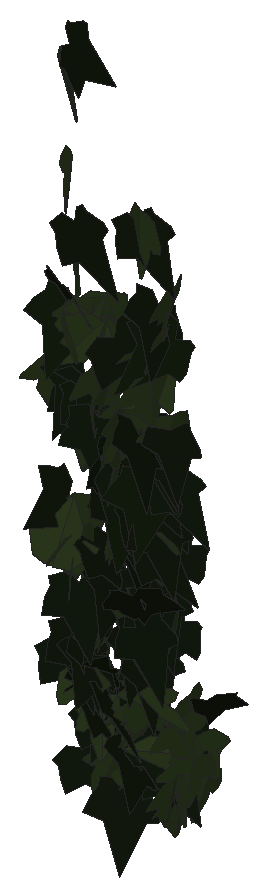
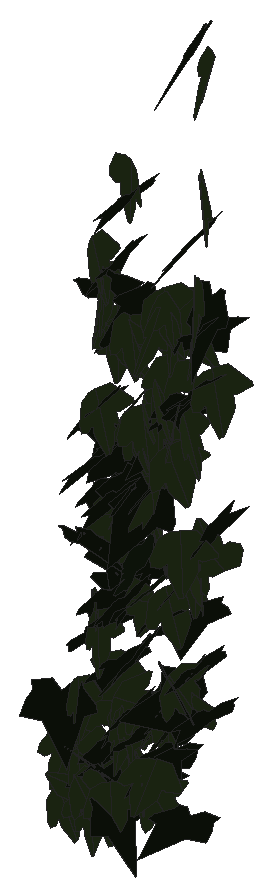
# SketchUp Ruby script. Lengths in inches.
U = 1.inch
M = Sketchup.active_model
def pt(a) = Geom::Point3d.new(a.map { |v| v * U })
def face(e, loops, mat)
  f = e.add_face(loops[0].map { |a| pt(a) })
  loops[1..].each { |l| e.add_face(l.map { |a| pt(a) }).erase! }
  f.material = f.back_material = mat if mat
  f
end
# faces: each face lists its corners as indices into pts; further lists are holes
def faces(e, pts, list, mat = nil) = list.each { |f| face(e, (f[0].is_a?(Array) ? f : [f]).map { |l| l.map { |i| pts[i] } }, mat) }
# xy, xz, yz: faces in a plane at the given z, y or x. An outline is a flat list of corners, or four numbers for a rectangle; further outlines are holes
def ring(l) = l.size == 4 ? [[l[0], l[1]], [l[2], l[1]], [l[2], l[3]], [l[0], l[3]]] : l.each_slice(2).to_a
def flat(e, list, mat, &to3) = list.each { |f| face(e, (f[0].is_a?(Array) ? f : [f]).map { |l| ring(l).map { |u, v| to3.(u, v) } }, mat) }
def xy(e, z, list, mat = nil) = flat(e, list, mat) { |x, y| [x, y, z] }
def xz(e, y, list, mat = nil) = flat(e, list, mat) { |x, z| [x, y, z] }
def yz(e, x, list, mat = nil) = flat(e, list, mat) { |y, z| [x, y, z] }
def lines(e, pts, list) = list.each { |a, b| e.add_line(pt(pts[a]), pt(pts[b])) }
# prism: a flat outline (further loops are holes) pulled along v
def prism(e, loops, v, mat = nil)
  f = face(e, loops, mat); d = Geom::Vector3d.new(v.map { |x| x * U })
  f.pushpull(f.normal.samedirection?(d) ? d.length : -d.length)
end
def box(e, o, s, mat = nil) = prism(e, [[o, [o[0] + s[0], o[1], o[2]], [o[0] + s[0], o[1] + s[1], o[2]], [o[0], o[1] + s[1], o[2]]]], [0, 0, s[2]], mat)
def at(x, y, z, deg = 0) = Geom::Transformation.translation(pt([x, y, z])) * Geom::Transformation.rotation(ORIGIN, Z_AXIS, deg.degrees)
def axes(o, x, y, z) = Geom::Transformation.new([*x, 0, *y, 0, *z, 0, *pt(o).to_a, 1])
def part(name) = M.definitions.add(name)
# library, detail: a bought-in or finely detailed component or shape, given as its bounding box
def library(name, o, s) = part(name).tap { |d| box(d.entities, o, s) }
def detail(e, o, s) = box(e.add_group.entities, o, s)
def put(e, d, t, mat = nil) = e.add_instance(d, t).tap { |i| i.material = mat if mat }
def group(e, t, mat = nil) = e.add_group.tap { |g| g.transformation = t; g.material = mat if mat }.entities
root = M.entities
M.materials.add("efeu1").color = [18, 25, 13]
M.materials.add("efeu2").color = [43, 57, 29]
c1 = part("ivyleaf_9")
p = [[1.54,2.16,1.25],[1.36,2.04,1.19],[-0.21,0.99,0.68],[-0.71,1.11,0.82],[-0.85,0.86,0.67],[-0.8,0.17,0.21],
  [-0.9,-0.01,0.1],[-0.67,-0.16,-0.02],[-0.08,-0.08,-0.05],[-0.03,-0.6,-0.4],[0.65,-0.88,-0.66],[0.83,-0.6,-0.49],
  [1.29,-0.42,-0.43],[1.8125,-0.07,-0.26],[1.21,0.44,0.15]]
faces(c1.entities,p,[[0,1,2,3,4,5,6,7,8,9,10,11,12,13,14]],"efeu1")
c2 = part("ivyleaf_10")
p = [[0,0.5,-0.03],[-0.0625,2.02,-0.43],[-0.19,2.01,-0.46],[-0.54,1.05,-0.29],[-0.52,0.625,-0.18],[-0.83,0.76,-0.28],
  [-1.16,0.64,-0.33],[-1.15,0.33,-0.24],[-0.77,-0.39,0.02],[-0.3,-0.51,0.16],[0.04,-0.48,0.23],[-0.02,2.01,-0.4375],
  [-0.06,2.01,-0.43],[0.04,-0.49,0.23],[0.67,-0.49,0.14],[1.38,0.36,-0.2],[1.375,0.51,-0.24],[0.81,0.65,-0.19],
  [0.62,0.59,-0.15],[0.6,1.09,-0.28],[0.5,1.23,-0.31]]
faces(c2.entities,p,[[0,1,2,3,4,5,6,7,8,9,10],[11,12,0,13,14,15,16,17,18,19,20]],"efeu2")
put(root,c1,axes([523.03,133.5,210.82],[0.21573,-0.75981,-0.367],[0.08957,0.39729,-0.76985],[0.83903,0.15295,0.17655]))
put(root,c2,axes([523.63,132.39,222.53],[-0.3306,-0.85871,0.06277],[-0.02819,-0.05641,-0.92013],[0.86054,-0.33174,-0.00602]))
put(root,c1,axes([523.49,133.05,216.98],[-0.21291,-0.48592,0.71831],[-0.21885,-0.6856,-0.52866],[0.83917,-0.30209,0.04437]))
put(root,c1,axes([523.875,132.32,225.51],[0.71123,0.0971,-0.62296],[-0.62829,0.0309,-0.7125],[-0.05254,0.94497,0.08731]))
put(root,c2,axes([523.84,133.06,226.16],[0.60515,-0.59939,-0.36822],[-0.0232,0.46845,-0.80067],[0.70308,0.53136,0.29052]))
put(root,c2,axes([523.79,132.78,229.89],[0.63105,-0.68924,-0.10856],[0.05514,0.19517,-0.91865],[0.69555,0.60985,0.17131]))
put(root,c1,axes([523.55,133.9,206.89],[0.0931,-0.46332,-0.70698],[0.16581,0.70745,-0.44179],[0.82885,-0.08948,0.16779]))
put(root,c1,axes([523.88,134.41,212.0625],[-0.6092,-0.01807,-0.6065],[0.60267,-0.11783,-0.60184],[-0.07046,-0.85152,0.09615]))
put(root,c1,axes([523.88,132.8125,224.51],[-0.36058,-0.84483,0.10318],[-0.00297,-0.11081,-0.91767],[0.85111,-0.35831,0.04051]))
put(root,c2,axes([524.15,133.57,216.76],[-0.68064,-0.54724,0.07313],[-0.04933,-0.05533,-0.87327],[0.5499,-0.68232,0.01217]))
put(root,c2,axes([524.09,133.18,221.02],[0.24465,-0.8658,0.02358],[0.00663,-0.02264,-0.8997],[0.8661,0.24474,0.00022]))
put(root,c2,axes([524.17,132.74,215.72],[-0.12082,-0.88019,-0.12853],[0.03912,0.12433,-0.88818],[0.88866,-0.12514,0.02163]))
put(root,c2,axes([524.11,132.16,234.07],[-0.61761,0.74402,-0.02898],[0.01411,-0.02596,-0.96694],[-0.74445,-0.61774,0.00572]))
put(root,c2,axes([523.95,131.97,215.53],[0.75966,0.48087,-0.2889],[0.23367,0.17089,0.89887],[0.51,-0.79457,0.01848]))
put(root,c2,axes([524.45,131.98,224.37],[-0.4241,0.60088,0.59974],[-0.34304,0.49196,-0.73547],[-0.77658,-0.54546,-0.00265]))
put(root,c1,axes([523.9375,133.02,211.93],[0.17442,-0.9103,-0.19992],[-0.03601,0.19666,-0.92686],[0.9313,0.1781,0.00161]))
put(root,c2,axes([523.92,132.89,214.72],[0.14046,-0.48894,-0.7946],[0.31519,-0.73145,0.5058],[-0.87813,-0.34075,0.05444]))
put(root,c2,axes([524.47,133.62,219.87],[-0.38353,-0.75266,0.2885],[-0.05201,-0.29572,-0.84064],[0.80438,-0.378,0.0832]))
put(root,c2,axes([524.3,133.57,211.45],[-0.14596,-0.73088,0.51134],[0.15822,-0.53114,-0.71401],[0.87785,-0.02579,0.21371]))
put(root,c2,axes([524.24,134.94,208.83],[-0.58602,-0.53911,-0.26307],[0.28378,0.07486,-0.78557],[0.5285,-0.63798,0.13012]))
put(root,c2,axes([524.51,133.6875,214.63],[-0.37975,-0.78041,0.18899],[-0.00526,-0.20663,-0.86385],[0.80295,-0.37044,0.08372]))
put(root,c1,axes([524.28,132.9375,221.98],[-0.29103,-0.80059,0.32103],[-0.03777,-0.32666,-0.84886],[0.86173,-0.28469,0.07122]))
put(root,c1,axes([524.19,132.875,213.875],[-0.08988,-0.83891,-0.33722],[0.01227,0.33772,-0.84342],[0.90407,-0.08799,-0.02208]))
put(root,c1,axes([524.43,134.62,208.91],[-0.35834,-0.76013,0.12156],[-0.02551,-0.12228,-0.83987],[0.76936,-0.3581,0.02877]))
put(root,c1,axes([524.52,132.0625,235.11],[0.54818,-0.2604,-0.75335],[-0.52182,0.57391,-0.57807],[0.60253,0.73393,0.18475]))
put(root,c1,axes([524.28,133.43,211.31],[0.19519,-0.80873,0.27072],[0.07608,-0.2601,-0.83186],[0.84944,0.20913,0.01229]))
put(root,c1,axes([524.43,132.83,221.9],[-0.06855,-0.82223,-0.38597],[0.00649,0.38661,-0.82476],[0.90829,-0.06481,-0.02324]))
put(root,c1,axes([524.25,132.625,227.875],[0.51084,-0.80431,-0.34052],[-0.08083,0.34925,-0.94621],[0.86967,0.50491,0.11207]))
put(root,c1,axes([524.35,133.68,208.99],[0.20424,-0.55464,-0.62506],[0.05035,0.65046,-0.56073],[0.83414,0.09654,0.18689]))
put(root,c2,axes([524.3125,132.73,210.45],[0.78011,0.12833,0.4222],[0.41328,0.08811,-0.7904],[-0.15468,0.88265,0.01752]))
put(root,c2,axes([524.83,133.98,207.21],[-0.1383,-0.75555,0.39257],[0.0079,-0.39884,-0.76482],[0.85141,-0.11903,0.07086]))
put(root,c2,axes([525.13,132.38,224.23],[0.68066,0.26824,-0.58825],[-0.60396,-0.04096,-0.71752],[-0.23069,0.8987,0.14287]))
put(root,c1,axes([524.3,132.74,210.31],[0.52021,0.2606,0.68132],[0.58923,0.3432,-0.58116],[-0.43002,0.78551,0.02789]))
put(root,c2,axes([525.1,132.54,220.4],[0.05653,-0.12748,-0.93577],[-0.25124,0.90163,-0.138],[0.91038,0.25674,0.02002]))
put(root,c1,axes([524.58,133.15,211.19],[-0.16461,-0.73641,0.45049],[0.10289,-0.47207,-0.7341],[0.85712,-0.08476,0.17464]))
put(root,c2,axes([525.04,132.54,225.08],[-0.62002,-0.70202,0.08547],[-0.05615,-0.06445,-0.93662],[0.70497,-0.62256,0.00058]))
put(root,c1,axes([524.61,132.83,221.49],[0.19262,-0.84865,-0.26493],[0.04034,0.27914,-0.86484],[0.88813,0.17138,0.09674]))
put(root,c2,axes([525.09,134.54,208.64],[0.43015,-0.67352,-0.26046],[-0.07574,0.25942,-0.79591],[0.71815,0.43078,0.07207]))
put(root,c2,axes([525.22,132.85,224.3125],[-0.8552,0.38411,0.00997],[-0.10854,-0.21816,-0.90534],[-0.36859,-0.82697,0.24346]))
put(root,c2,axes([525.03,133.28,219.85],[-0.27148,0.82044,-0.30303],[0.00378,-0.31619,-0.85946],[-0.87461,-0.25604,0.09034]))
put(root,c2,axes([525.18,133.28,222.01],[0.30272,-0.86255,-0.00942],[-0.00033,0.00987,-0.91413],[0.8626,0.30271,0.00296]))
put(root,c2,axes([525.29,132.82,225.18],[-0.51357,-0.7449,0.21719],[-0.04188,-0.23346,-0.89975],[0.77479,-0.50638,0.09533]))
put(root,c1,axes([524.6875,133.13,215.5625],[0.5326,-0.64442,-0.27208],[-0.01428,0.33188,-0.81402],[0.69936,0.49754,0.19058]))
put(root,c1,axes([524.92,132.63,209.88],[0.63151,-0.51188,-0.38719],[-0.26374,0.28825,-0.81123],[0.58513,0.68237,0.05223]))
put(root,c2,axes([525.23,132.69,222.55],[-0.3423,-0.77182,-0.36409],[0.16124,0.32673,-0.84421],[0.83802,-0.37812,0.01371]))
put(root,c1,axes([525,133.69,214.04],[-0.01519,-0.77389,0.42218],[0.01894,-0.42243,-0.77367],[0.88135,-0.00426,0.0239]))
put(root,c2,axes([525.29,132.77,209.625],[0.45676,0.73847,-0.0626],[-0.0381,-0.05004,-0.86829],[-0.74014,0.45831,0.00606]))
put(root,c2,axes([525.39,133.14,224.45],[0.0886,-0.64485,-0.65367],[0.1406,0.65849,-0.63054],[0.90738,-0.03907,0.16153]))
put(root,c2,axes([525.4,133.49,218.07],[-0.08307,0.85943,-0.28009],[-0.02683,-0.28349,-0.86191],[-0.90353,-0.0706,0.05135]))
put(root,c1,axes([525.3125,132.48,220.83],[-0.10146,-0.87954,-0.25125],[0.00607,0.25213,-0.8851],[0.9147,-0.09924,-0.022]))
put(root,c2,axes([525.78,132.88,216.68],[0.49406,-0.67286,-0.31123],[-0.20426,0.23599,-0.83444],[0.71266,0.53411,-0.0234]))
put(root,c2,axes([525.81,133.4,220.85],[-0.43796,-0.78933,0.05645],[-0.02378,-0.05136,-0.90268],[0.79099,-0.43858,0.00412]))
put(root,c2,axes([525.88,133.19,220.61],[-0.81924,-0.34443,0.10191],[-0.08006,-0.07234,-0.888],[0.35016,-0.82238,0.03542]))
put(root,c1,axes([525.91,131.93,219.89],[0.0056,0.26119,-0.90162],[-0.57394,0.71442,0.2034],[0.74279,0.55005,0.16395]))
put(root,c1,axes([526.16,134.5,206.71],[-0.20807,0.75605,-0.28918],[0.09248,-0.27443,-0.78401],[-0.80417,-0.22718,-0.01533]))
put(root,c1,axes([525.8,133.14,217.95],[0.75241,0.5911,-0.06795],[-0.05293,-0.04262,-0.95682],[-0.59263,0.75427,-0.00081]))
put(root,c1,axes([525.46,132.6875,210.1875],[0.59051,-0.63107,0.1221],[0.07528,-0.09676,-0.8642],[0.63835,0.59519,-0.01104]))
put(root,c2,axes([526.13,134.74,207.18],[-0.50562,-0.66715,0.00749],[0.00439,-0.01273,-0.83703],[0.66718,-0.50551,0.01119]))
put(root,c1,axes([525.76,134.16,209.17],[-0.02041,-0.85712,0.0673],[0.00856,-0.06752,-0.8573],[0.85972,-0.01968,0.01013]))
put(root,c2,axes([525.98,132.79,221],[0.32254,-0.7633,0.37634],[0.13325,-0.3522,-0.82855],[0.84054,0.34874,-0.01307]))
put(root,c2,axes([526.18,133.88,210.32],[-0.09733,-0.42905,0.75789],[-0.02247,-0.76111,-0.43377],[0.87062,-0.06761,0.07353]))
put(root,c2,axes([525.9,133.01,219.58],[0.42169,-0.66619,0.47453],[0.26959,-0.39084,-0.78827],[0.77221,0.50024,0.01607]))
put(root,c1,axes([525.72,134.16,210.29],[0.34823,-0.76295,-0.24811],[-0.05508,0.2471,-0.83715],[0.80038,0.34895,0.05033]))
put(root,c2,axes([526.25,132.97,220.08],[-0.13041,-0.88121,0.04249],[-0.00823,-0.04174,-0.89081],[0.8822,-0.13066,-0.00203]))
put(root,c2,axes([526.22,133.53,209.7],[0.05641,-0.848,-0.17399],[0.00408,0.17461,-0.84973],[0.86565,0.05444,0.01534]))
put(root,c2,axes([526.19,133.95,209.58],[0.04514,-0.78293,-0.37668],[0.06182,0.37913,-0.78061],[0.86663,0.01374,0.0753]))
put(root,c2,axes([526.13,133.5625,206.97],[-0.0542,-0.63522,0.62819],[0.23889,-0.61674,-0.60302],[0.86085,0.13115,0.20689]))
put(root,c1,axes([525.84,132.58,218.18],[0.34782,-0.86169,-0.09061],[-0.026,0.08722,-0.9292],[0.86605,0.34869,0.0085]))
put(root,c1,axes([525.98,133.74,211.96],[0.05377,-0.80925,0.34041],[0.00719,-0.34063,-0.81091],[0.87791,0.05236,-0.01421]))
put(root,c2,axes([526.38,133.51,208.9],[-0.08237,-0.8522,-0.16457],[-0.00197,0.16549,-0.85599],[0.86794,-0.0805,-0.01756]))
put(root,c1,axes([525.93,133.65,215.25],[0.20812,-0.66904,0.55304],[0.2253,-0.50759,-0.69884],[0.83828,0.30253,0.05052]))
put(root,c2,axes([526.51,133.5,209.72],[-0.12342,-0.76625,0.4123],[0.0355,-0.42052,-0.77089],[0.86941,-0.09161,0.09001]))
put(root,c1,axes([526.13,133.98,214.27],[0.24094,-0.83446,-0.16753],[-0.01818,0.16902,-0.86806],[0.85091,0.23989,0.02889]))
put(root,c1,axes([526.32,132.77,206.63],[-0.21215,-0.90102,-0.1024],[0.02489,0.09934,-0.92566],[0.90648,-0.2136,0.00145]))
put(root,c1,axes([526.27,132.75,217.96],[-0.09042,-0.89353,0.13845],[0.03712,-0.14269,-0.89667],[0.90343,-0.08357,0.0507]))
put(root,c1,axes([526.48,132.99,217.76],[0.40897,-0.59364,-0.51117],[-0.26747,0.43617,-0.72054],[0.73632,0.48817,0.02218]))
put(root,c2,axes([526.09,132.96,213.66],[-0.18481,-0.00066,-0.86106],[0.83923,-0.19716,-0.17998],[-0.19263,-0.85832,0.042]))
put(root,c1,axes([526.35,133.08,208.0625],[0.05771,-0.76984,0.47996],[0.13291,-0.46857,-0.76755],[0.89742,0.1189,0.08281]))
put(root,c2,axes([526.91,132.66,223.66],[-0.2328,-0.89746,-0.00374],[-0.00346,0.00476,-0.92716],[0.89746,-0.23278,-0.00455]))
put(root,c2,axes([526.62,133.55,216.73],[0.58829,0.65833,0.0137],[0.03105,-0.00938,-0.88239],[-0.65774,0.58838,-0.0294]))
put(root,c1,axes([526.52,131.97,224.56],[0.17408,-0.44315,-0.83753],[0.00675,0.85211,-0.44946],[0.94752,0.07535,0.15708]))
put(root,c1,axes([526.58,133.78,211.68],[0.04501,-0.84877,-0.2057],[0.04469,0.20794,-0.84824],[0.8722,0.03314,0.05408]))
put(root,c1,axes([526.5625,133.93,217.99],[0.30843,-0.72583,-0.40656],[-0.02423,0.42558,-0.77817],[0.83159,0.2816,0.12811]))
put(root,c1,axes([526.68,133.87,208.58],[-0.01011,-0.79231,-0.36591],[0.00947,0.36581,-0.79236],[0.87267,-0.01315,0.00435]))
put(root,c1,axes([526.57,133.48,211.25],[0.19098,-0.80234,0.30186],[0.11465,-0.28258,-0.82362],[0.84955,0.21851,0.04329]))
put(root,c2,axes([527.37,134.06,208.03],[-0.01468,0.28991,0.81988],[-0.36205,-0.74759,0.25787],[0.79068,-0.33694,0.1333]))
put(root,c2,axes([527.08,134.1,213],[0.03949,-0.84868,-0.1854],[0.03396,0.18696,-0.84858],[0.86803,0.03129,0.04163]))
put(root,c2,axes([527.08,135.09,207.34],[0.05338,-0.76144,0.32186],[0.07422,-0.31681,-0.76181],[0.82333,0.07793,0.04781]))
put(root,c2,axes([527.3,132.37,229.13],[-0.85077,0.44371,-0.02949],[-0.09882,-0.2507,-0.92138],[-0.43357,-0.81353,0.26786]))
put(root,c2,axes([527.5,132.73,223.2],[0.76705,0.05981,-0.52265],[-0.52563,0.04982,-0.76572],[-0.02125,0.92685,0.07488]))
put(root,c1,axes([527.75,134.71,208.21],[-0.80607,0.22484,0.13716],[-0.174,-0.1231,-0.82078],[-0.19771,-0.80834,0.16315]))
put(root,c2,axes([527.3,134.29,206.22],[-0.06685,-0.82828,-0.08372],[0.02719,0.08177,-0.83072],[0.83206,-0.06922,0.02042]))
put(root,c1,axes([526.94,133.64,214.06],[0.01772,-0.83507,-0.3101],[0.00847,0.31031,-0.83514],[0.89074,0.01367,0.01411]))
put(root,c1,axes([526.91,134.17,207.58],[0.11628,-0.67687,-0.5282],[0.01812,0.53484,-0.68139],[0.85838,0.0804,0.08593]))
put(root,c1,axes([527.27,131.98,214.93],[0.64491,0.6361,-0.27839],[-0.19316,-0.20059,-0.90581],[-0.66694,0.67318,-0.00685]))
put(root,c1,axes([526.83,132.86,228.67],[0.31331,-0.83809,-0.26319],[0.05464,0.29748,-0.88224],[0.87675,0.28096,0.14903]))
put(root,c1,axes([526.86,132.74,220.59],[0.23168,-0.90044,0.27415],[0.06342,-0.26676,-0.92975],[0.93911,0.24016,-0.00484]))
put(root,c1,axes([527.26,134.55,212.83],[-0.31746,-0.70125,0.37246],[-0.08134,-0.3703,-0.7665],[0.78985,-0.31998,0.07077]))
put(root,c1,axes([526.91,132.93,219.37],[-0.23737,-0.37457,-0.79739],[0.53661,0.59349,-0.43853],[0.6987,-0.58305,0.06589]))
put(root,c2,axes([527.5,133.61,220.95],[-0.19179,-0.87342,0.1034],[-0.00221,-0.10535,-0.894],[0.87952,-0.19072,0.0203]))
put(root,c2,axes([527.53,134.55,207.87],[0.07285,-0.81952,-0.23105],[-0.01348,0.23075,-0.82272],[0.85136,0.07378,0.00674]))
put(root,c1,axes([527.33,132.71,218.89],[-0.40992,-0.78959,-0.16269],[0.09214,0.13543,-0.88945],[0.8009,-0.41971,0.01906]))
put(root,c2,axes([527.4,132.45,216.93],[-0.845,-0.14706,-0.20845],[0.21119,0.00133,-0.85703],[0.1431,-0.87033,0.03391]))
put(root,c2,axes([527.03,134.66,206.89],[0.37163,0.21744,-0.72133],[0.59869,0.40303,0.42994],[0.45735,-0.70427,0.02333]))
put(root,c2,axes([527.56,133.77,213.45],[0.45464,-0.68958,-0.30711],[-0.04025,0.33586,-0.81371],[0.7538,0.43384,0.14178]))
put(root,c2,axes([527.26,132.53,210.53],[-0.48423,-0.27206,-0.68845],[0.61064,0.31822,-0.55526],[0.41844,-0.77921,0.01361]))
put(root,c2,axes([527.62,133.74,207.33],[-0.7039,0.42463,-0.15601],[0.08271,-0.16289,-0.81655],[-0.44475,-0.70234,0.09506]))
put(root,c1,axes([527.89,134.125,216.11],[-0.83642,-0.22783,-0.10408],[0.12107,-0.05016,-0.86323],[0.21927,-0.84138,0.07964]))
put(root,c1,axes([527.33,132.48,213.53],[-0.45635,-0.30959,-0.73877],[0.63913,0.37179,-0.55061],[0.48285,-0.78473,0.03059]))
put(root,c2,axes([527.79,135.16,206.72],[-0.1033,-0.79687,0.19354],[0.00215,-0.19533,-0.8031],[0.82003,-0.09987,0.02649]))
put(root,c2,axes([527.76,133.15,224.83],[0.40192,-0.66154,-0.4994],[-0.02161,0.54646,-0.74127],[0.82859,0.33514,0.22291]))
put(root,c2,axes([527.8,133.29,207.24],[0.04653,-0.83337,-0.04496],[0.01169,0.04568,-0.83454],[0.8345,0.04583,0.01419]))
put(root,c2,axes([527.83,132.1875,223.3],[-0.28176,-0.95589,-0.13853],[0.03785,0.13326,-0.99655],[0.96514,-0.28429,-0.00135]))
put(root,c2,axes([527.9,134.11,210.22],[0.05391,-0.82425,-0.20479],[0.02839,0.20683,-0.82501],[0.84883,0.04543,0.0406]))
put(root,c2,axes([527.9375,133.15,226.3],[0.21442,-0.89774,-0.02066],[-0.001,0.021,-0.92299],[0.89798,0.21439,0.0039]))
put(root,c1,axes([527.6,132.83,225.74],[0.04213,-0.89919,0.24159],[-0.01129,-0.24232,-0.89991],[0.93101,0.03775,-0.02185]))
put(root,c2,axes([527.9375,133.55,209.42],[-0.3677,-0.72469,-0.32601],[0.13056,0.29924,-0.81244],[0.78384,-0.3898,-0.01761]))
put(root,c1,axes([527.61,133.66,220.68],[0.09695,-0.88731,0.07237],[0.01073,-0.07163,-0.89259],[0.89019,0.0975,0.00287]))
put(root,c1,axes([528.3,132.7,224.85],[-0.82465,-0.3673,0.14155],[-0.1282,-0.06006,-0.90275],[0.37217,-0.83455,0.00267]))
put(root,c2,axes([528.04,132.47,224.99],[0.20752,-0.8249,-0.38584],[0.04225,0.40402,-0.84105],[0.90969,0.16941,0.12708]))
put(root,c1,axes([527.72,132.77,217.61],[0.07359,-0.87197,-0.23761],[-0.02331,0.23648,-0.87507],[0.90347,0.07712,-0.00322]))
put(root,c1,axes([527.59,133.56,218.83],[0.3262,-0.77871,-0.29159],[0.08121,0.34157,-0.82132],[0.82754,0.27344,0.19554]))
put(root,c1,axes([527.64,132.46,216.85],[0.45274,-0.65292,-0.42802],[-0.05505,0.46685,-0.77039],[0.77877,0.41258,0.19437]))
put(root,c1,axes([528.3125,134.5625,210.16],[0.24339,0.77377,-0.27334],[-0.21424,-0.2153,-0.80026],[-0.79217,0.29597,0.13245]))
put(root,c2,axes([528.2,133.9,207.93],[-0.38129,-0.78406,0.03692],[-0.01079,-0.03581,-0.87184],[0.78486,-0.3814,0.00595]))
put(root,c2,axes([528.06,134.47,208.49],[-0.5106,-0.61685,-0.28483],[0.19236,0.21048,-0.80065],[0.65164,-0.54548,0.01316]))
